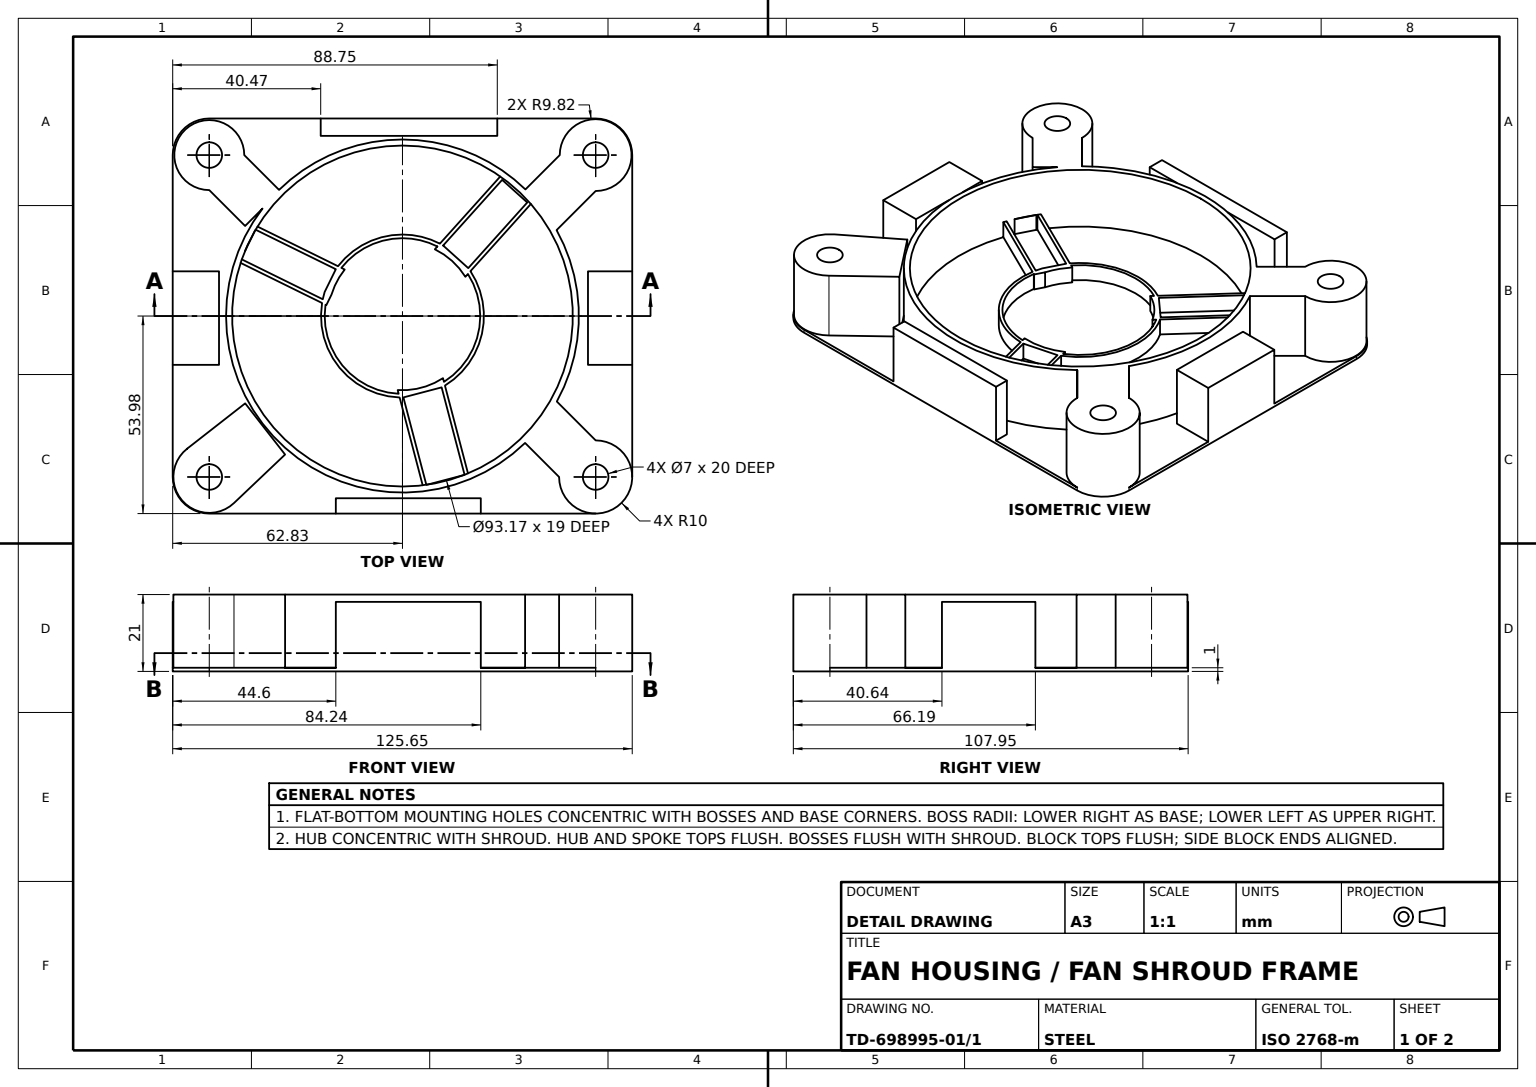
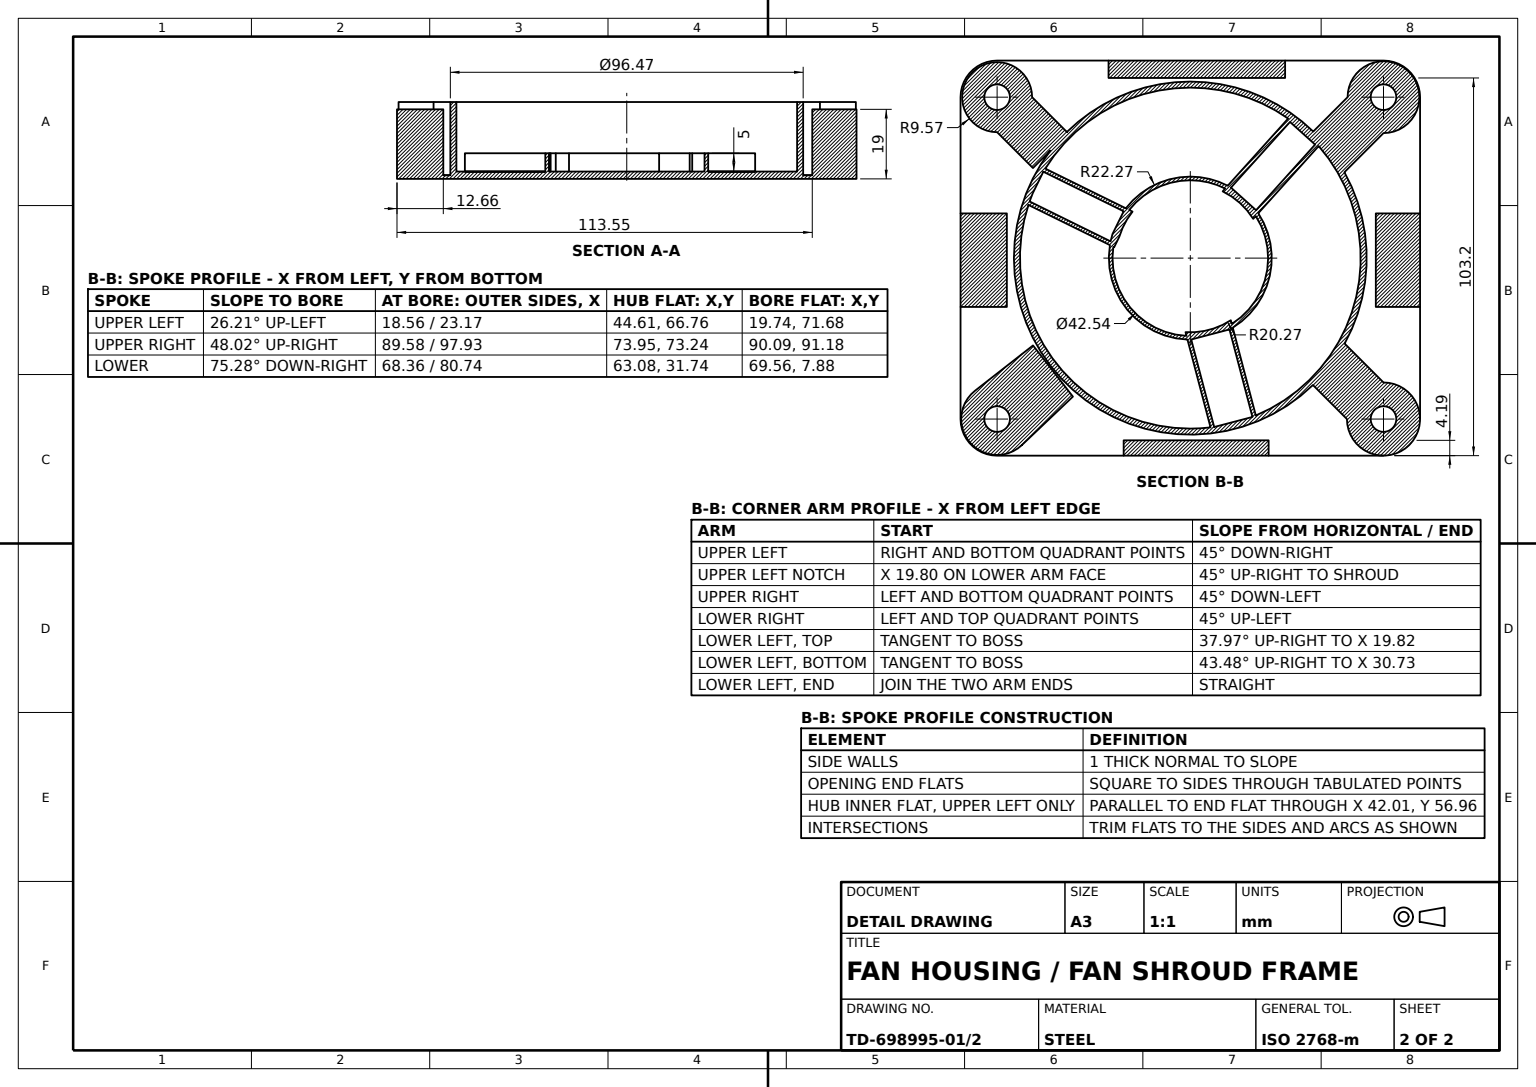
solid
v1 (0,7,-21.270645)
v2 (0,2,-21.270645)
e1 v1 v2 LINE
v3 (9.545019,2,-19.00876)
e2 v3 v2 CIRCLE(AX(P(0,2,0),D(0,1,0),D(0,0,1)),21.270645)
v4 (9.545019,7,-19.00876)
e3 v3 v4 LINE
e4 v4 v1 CIRCLE(AX(P(0,7,0),D(0,1,0),D(0,0,1)),21.270645)
face CYL(AX(P(0,7,0),D(0,-1,0),D(0,0,-1)),21.270645) rev [e1 -e2 e3 e4]
v5 (33.621716,21,-34.589177)
v6 (33.621716,1,-34.589177)
e5 v5 v6 LINE
v7 (43.007539,21,-43.975)
e6 v7 v5 LINE
v8 (43.007539,1,-43.975)
e7 v7 v8 LINE
e8 v8 v6 LINE
face PLANE(AX(P(-0.48373,21,-0.48373),D(0.707106781,0,0.707106781),D(0.707106781,0,-0.707106781))) rev [-e5 -e6 e7 e8]
v9 (52.826203,1,-53.975)
v10 (52.826203,0,-53.975)
e9 v9 v10 LINE
v11 (-52.826203,0,-53.975)
e10 v10 v11 LINE
v12 (-52.826203,1,-53.975)
e11 v12 v11 LINE
v13 (-22.357204,1,-53.975)
e12 v13 v12 LINE
v14 (-22.357204,19,-53.975)
e13 v14 v13 LINE
v15 (25.926841,19,-53.975)
e14 v15 v14 LINE
v16 (25.926841,1,-53.975)
e15 v15 v16 LINE
e16 v9 v16 LINE
face PLANE(AX(P(-52.826203,1,-53.975),D(0,0,1),D(1,0,0))) rev [e9 e10 -e11 -e12 -e13 -e14 e15 -e16]
v17 (-21.7948,2,-4.579116)
v18 (-21.7948,7,-4.579116)
e17 v17 v18 LINE
v19 (-21.281374,7,-6.563897)
e18 v19 v18 CIRCLE(AX(P(0,7,0),D(0,1,0),D(1,0,0)),22.270645)
v20 (-21.281374,2,-6.563897)
e19 v19 v20 LINE
e20 v20 v17 CIRCLE(AX(P(0,2,0),D(0,1,0),D(1,0,0)),22.270645)
face CYL(AX(P(0,7,0),D(0,-1,0),D(0,0,-1)),22.270645) [e17 -e18 e19 e20]
v21 (-32.095624,1,37.844091)
v22 (-46.070336,1,51.098182)
e21 v21 v22 LINE
v23 (-32.095624,21,37.844091)
e22 v23 v21 LINE
v24 (-46.070336,21,51.098182)
e23 v23 v24 LINE
e24 v24 v22 LINE
face PLANE(AX(P(3.696574,21,3.897556),D(0.688151966,0,0.725566587),D(0.725566587,0,-0.688151966))) [-e21 -e22 e23 e24]
v25 (-43.008797,21,23.860209)
v26 (-43.008797,1,23.860209)
e25 v25 v26 LINE
v27 (-58.866196,1,36.235495)
e26 v27 v26 LINE
v28 (-58.866196,21,36.235495)
e27 v28 v27 LINE
e28 v28 v25 LINE
face PLANE(AX(P(-4.706752,21,-6.031121),D(-0.615233142,0,-0.788345217),D(-0.788345217,0,0.615233142))) [e25 -e26 -e27 e28]
v29 (-1.307728,7,20.228418)
v30 (-1.307728,2,20.228418)
e29 v29 v30 LINE
v31 (-1.040622,2,21.245175)
e30 v30 v31 LINE
v32 (-1.040622,7,21.245175)
e31 v31 v32 LINE
e32 v29 v32 LINE
face PLANE(AX(P(-6.194325,7,1.627275),D(0.967182465,0,-0.254082822),D(-0.254082822,0,-0.967182465))) rev [e29 e30 e31 -e32]
v33 (-43.937779,7,-15.47732)
e33 v18 v33 LINE
v34 (-43.937779,2,-15.47732)
e34 v17 v34 LINE
e35 v33 v34 LINE
face PLANE(AX(P(-2.435731,7,4.94892),D(-0.441587655,0,0.897218113),D(0.897218113,0,0.441587655))) rev [-e33 -e17 e34 -e35]
v35 (-40.168907,7,-23.590988)
v36 (-40.168907,2,-23.590988)
e36 v35 v36 LINE
v37 (-18.218296,2,-12.787462)
e37 v37 v36 LINE
v38 (-18.218296,7,-12.787462)
e38 v38 v37 LINE
e39 v38 v35 LINE
face PLANE(AX(P(1.513837,7,-3.075815),D(-0.441587655,0,0.897218113),D(0.897218113,0,0.441587655))) [e36 -e37 -e38 e39]
v39 (-62.826203,1,13.339172)
v40 (-62.826203,1,43.975)
e40 v39 v40 LINE
v41 (-52.826203,1,53.975)
e41 v40 v41 CIRCLE(AX(P(-52.826203,1,43.975),D(0,1,0),D(0,0,1)),10)
v42 (-18.223939,1,53.975)
e42 v41 v42 LINE
v43 (-18.223939,1,49.787051)
e43 v43 v42 LINE
v44 (21.417826,1,49.787051)
e44 v44 v43 LINE
v45 (21.417826,1,53.975)
e45 v45 v44 LINE
v46 (52.826203,1,53.975)
e46 v45 v46 LINE
v47 (42.826203,1,43.975)
e47 v47 v46 CIRCLE(AX(P(52.826203,1,43.975),D(0,1,0),D(0,0,1)),10)
v48 (33.529642,1,34.678439)
e48 v47 v48 LINE
v49 (-38.265553,1,-29.369685)
e49 v49 v48 CIRCLE(AX(P(0,1,0),D(0,1,0),D(0,0,1)),48.237237)
v50 (-43.027328,1,-24.60791)
e50 v50 v49 LINE
v51 (-52.826203,1,-34.406784)
e51 v51 v50 LINE
v52 (-52.826203,1,-53.543216)
e52 v52 v51 CIRCLE(AX(P(-52.826203,1,-43.975),D(0,1,0),D(0,0,1)),9.568216)
v53 (-43.257987,1,-43.975)
e53 v53 v52 CIRCLE(AX(P(-52.826203,1,-43.975),D(0,1,0),D(0,0,1)),9.568216)
v54 (-33.748486,1,-34.465499)
e54 v53 v54 LINE
v55 (0,1,-48.237237)
e55 v55 v54 CIRCLE(AX(P(0,1,0),D(0,1,0),D(0,0,1)),48.237237)
e56 v6 v55 CIRCLE(AX(P(0,1,0),D(0,1,0),D(0,0,1)),48.237237)
v56 (52.826203,1,-53.793663)
e57 v56 v8 CIRCLE(AX(P(52.826203,1,-43.975),D(0,1,0),D(0,0,1)),9.818663)
v57 (52.826203,1,-34.156337)
e58 v57 v56 CIRCLE(AX(P(52.826203,1,-43.975),D(0,1,0),D(0,0,1)),9.818663)
v58 (42.141556,1,-23.47169)
e59 v57 v58 LINE
v59 (42.20629,1,23.355087)
e60 v59 v58 CIRCLE(AX(P(0,1,0),D(0,1,0),D(0,0,1)),48.237237)
v60 (52.826203,1,33.975)
e61 v60 v59 LINE
v61 (62.826203,1,43.975)
e62 v61 v60 CIRCLE(AX(P(52.826203,1,43.975),D(0,1,0),D(0,0,1)),10)
v62 (62.826203,1,13.339172)
e63 v61 v62 LINE
v63 (50.726429,1,13.339172)
e64 v63 v62 LINE
v64 (50.726429,1,-12.211918)
e65 v64 v63 LINE
v65 (62.826203,1,-12.211918)
e66 v65 v64 LINE
v66 (62.826203,1,-43.975)
e67 v65 v66 LINE
e68 v66 v9 CIRCLE(AX(P(52.826203,1,-43.975),D(0,1,0),D(0,0,1)),10)
v67 (25.926841,1,-49.223424)
e69 v67 v16 LINE
v68 (-22.357204,1,-49.223424)
e70 v68 v67 LINE
e71 v13 v68 LINE
v69 (-62.826203,1,-43.975)
e72 v12 v69 CIRCLE(AX(P(-52.826203,1,-43.975),D(0,1,0),D(0,0,-1)),10)
v70 (-62.826203,1,-12.211918)
e73 v69 v70 LINE
v71 (-50.162802,1,-12.211918)
e74 v71 v70 LINE
v72 (-50.162802,1,13.339172)
e75 v72 v71 LINE
e76 v39 v72 LINE
e77 v27 v22 CIRCLE(AX(P(-52.826203,1,43.975),D(0,1,0),D(0,0,1)),9.817406)
e78 v26 v21 LINE
face PLANE(AX(P(52.826203,1,43.975),D(0,-1,0),D(0,0,-1))) rev [e40 e41 e42 -e43 -e44 -e45 e46 -e47 e48 -e49 -e50 -e51 -e52 -e53 e54 -e55 -e56 -e8 -e57 -e58 e59 -e60 -e61 -e62 e63 -e64 -e65 -e66 e67 e68 e16 -e69 -e70 -e71 e12 e72 e73 -e74 -e75 -e76] [-e77 e26 e78 e21]
v73 (-52.826203,1,47.475)
v74 (-52.826203,1,40.475)
e79 v73 v74 CIRCLE(AX(P(-52.826203,1,43.975),D(0,1,0),D(0,0,1)),3.5)
e80 v74 v73 CIRCLE(AX(P(-52.826203,1,43.975),D(0,1,0),D(0,0,1)),3.5)
face PLANE(AX(P(52.826203,1,43.975),D(0,-1,0),D(0,0,-1))) rev [e79 e80]
v75 (52.826203,1,40.475)
v76 (52.826203,1,47.475)
e81 v75 v76 CIRCLE(AX(P(52.826203,1,43.975),D(0,1,0),D(0,0,1)),3.5)
v77 (52.826203,21,40.475)
e82 v77 v75 LINE
v78 (52.826203,21,47.475)
e83 v77 v78 CIRCLE(AX(P(52.826203,21,43.975),D(0,1,0),D(0,0,1)),3.5)
e84 v78 v76 LINE
face CYL(AX(P(52.826203,21,43.975),D(0,-1,0),D(0,0,-1)),3.5) rev [-e81 -e82 e83 e84]
v79 (11.080922,7,16.973868)
v80 (11.080922,2,16.973868)
e85 v79 v80 LINE
e86 v30 v80 CIRCLE(AX(P(0,2,0),D(0,1,0),D(1,0,0)),20.270645)
e87 v29 v79 CIRCLE(AX(P(0,7,0),D(0,1,0),D(1,0,0)),20.270645)
face CYL(AX(P(0,7,0),D(0,-1,0),D(0,0,-1)),20.270645) rev [e85 -e86 -e29 e87]
v81 (-40.311639,2,-23.346255)
e88 v36 v81 CIRCLE(AX(P(0,2,0),D(0,1,0),D(0,0,1)),46.584073)
v82 (-39.651388,7,-24.450834)
e89 v35 v82 CIRCLE(AX(P(0,7,0),D(0,-1,0),D(0,0,1)),46.584073)
v83 (-39.651388,2,-24.450834)
e90 v83 v82 LINE
v84 (0,2,-46.584073)
e91 v84 v83 CIRCLE(AX(P(0,2,0),D(0,1,0),D(0,0,1)),46.584073)
v85 (0,21,-46.584073)
e92 v84 v85 LINE
v86 (0,21,46.584073)
e93 v85 v86 CIRCLE(AX(P(0,21,0),D(0,1,0),D(0,0,1)),46.584073)
v87 (0,2,46.584073)
e94 v87 v86 LINE
v88 (-44.262515,2,-14.52259)
e95 v88 v87 CIRCLE(AX(P(0,2,0),D(0,1,0),D(0,0,1)),46.584073)
v89 (-44.262515,7,-14.52259)
e96 v88 v89 LINE
e97 v89 v33 CIRCLE(AX(P(0,7,0),D(0,-1,0),D(0,0,1)),46.584073)
v90 (-43.08972,2,-17.701747)
e98 v90 v34 CIRCLE(AX(P(0,2,0),D(0,1,0),D(0,0,1)),46.584073)
v91 (-43.08972,7,-17.701747)
e99 v91 v90 LINE
v92 (-40.311639,7,-23.346255)
e100 v91 v92 CIRCLE(AX(P(0,7,0),D(0,-1,0),D(0,0,1)),46.584073)
e101 v92 v81 LINE
face CYL(AX(P(0,2,0),D(0,1,0),D(0,0,1)),46.584073) rev [-e88 -e36 e89 -e90 -e91 e92 e93 -e94 -e95 e96 e97 e35 -e98 -e99 e100 e101]
v93 (18.590913,2,-12.262119)
v94 (18.590913,7,-12.262119)
e102 v93 v94 LINE
v95 (35.107613,2,-30.619134)
e103 v93 v95 LINE
v96 (35.107613,7,-30.619134)
e104 v95 v96 LINE
e105 v94 v96 LINE
face PLANE(AX(P(4.176783,7,3.758055),D(-0.743387039,0,-0.668861503),D(-0.668861503,0,0.743387039))) rev [-e102 e103 e104 -e105]
v97 (17.203804,7,-10.720456)
v98 (17.203804,2,-10.720456)
e106 v97 v98 LINE
v99 (17.898585,2,-11.49265)
e107 v98 v99 LINE
v100 (17.898585,7,-11.49265)
e108 v99 v100 LINE
e109 v97 v100 LINE
face PLANE(AX(P(4.176783,7,3.758055),D(-0.743387039,0,-0.668861503),D(-0.668861503,0,0.743387039))) rev [e106 e107 e108 -e109]
v101 (10.237348,2,-19.778229)
v102 (10.237348,7,-19.778229)
e110 v101 v102 LINE
v103 (0,2,-22.270645)
e111 v101 v103 CIRCLE(AX(P(0,2,0),D(0,1,0),D(1,0,0)),22.270645)
v104 (0,7,-22.270645)
e112 v104 v103 LINE
e113 v102 v104 CIRCLE(AX(P(0,7,0),D(0,1,0),D(1,0,0)),22.270645)
face CYL(AX(P(0,7,0),D(0,-1,0),D(0,0,-1)),22.270645) [-e110 e111 -e112 -e113]
v105 (-43.027328,21,-24.60791)
e114 v105 v50 LINE
v106 (-52.826203,21,-34.406784)
e115 v106 v105 LINE
e116 v106 v51 LINE
face PLANE(AX(P(-9.209709,21,9.209709),D(0.707106781,0,-0.707106781),D(-0.707106781,0,-0.707106781))) rev [-e114 -e115 e116 e51]
v107 (-21.984596,7,-3.557972)
e117 v107 v89 LINE
v108 (-0.774768,7,22.257164)
e118 v107 v108 CIRCLE(AX(P(0,7,0),D(0,1,0),D(1,0,0)),22.270645)
v109 (5.529493,7,46.254735)
e119 v108 v109 LINE
v110 (6.529144,7,46.124247)
e120 v110 v109 CIRCLE(AX(P(0,7,0),D(0,-1,0),D(0,0,1)),46.584073)
v111 (0.254083,7,22.237827)
e121 v111 v110 LINE
v112 (10.708369,7,19.491443)
e122 v111 v112 LINE
v113 (16.98343,7,43.377863)
e123 v112 v113 LINE
v114 (17.918143,7,43.000186)
e124 v114 v113 CIRCLE(AX(P(0,7,0),D(0,-1,0),D(0,0,1)),46.584073)
v115 (11.613882,7,19.002615)
e125 v115 v114 LINE
e126 v115 v94 CIRCLE(AX(P(0,7,0),D(0,1,0),D(1,0,0)),22.270645)
v116 (26.754047,7,-38.135243)
e127 v116 v96 CIRCLE(AX(P(0,7,0),D(0,-1,0),D(0,0,1)),46.584073)
e128 v102 v116 LINE
v117 (-17.627231,7,-13.611111)
e129 v104 v117 CIRCLE(AX(P(0,7,0),D(0,1,0),D(1,0,0)),22.270645)
e130 v117 v82 LINE
e131 v19 v38 LINE
v118 (-15.792502,7,-12.708105)
v119 (-19.415279,7,-5.826317)
e132 v118 v119 CIRCLE(AX(P(0,7,0),D(0,1,0),D(1,0,0)),20.270645)
v120 (-16.710846,7,-13.16009)
e133 v118 v120 LINE
e134 v1 v120 CIRCLE(AX(P(0,7,0),D(0,1,0),D(0,0,1)),21.270645)
v121 (8.850238,7,-18.236566)
e135 v121 v4 LINE
e136 v97 v121 CIRCLE(AX(P(0,7,0),D(0,1,0),D(1,0,0)),20.270645)
v122 (11.348029,7,17.990625)
e137 v122 v100 CIRCLE(AX(P(0,7,0),D(0,1,0),D(0,0,1)),21.270645)
e138 v79 v122 LINE
v123 (-21.044247,7,-3.095157)
e139 v123 v32 CIRCLE(AX(P(0,7,0),D(0,1,0),D(0,0,1)),21.270645)
v124 (-20.815015,7,-2.982334)
e140 v124 v123 LINE
e141 v124 v119 LINE
v125 (27.258813,7,-37.201174)
v126 (34.125605,7,-31.022787)
e142 v125 v126 LINE
v127 (17.989939,7,-13.089261)
e143 v127 v126 LINE
v128 (11.123147,7,-19.267648)
e144 v128 v127 LINE
e145 v128 v125 LINE
face PLANE(AX(P(0,7,0),D(0,1,0),D(0,0,1))) [-e117 e118 e119 -e120 -e121 e122 e123 -e124 -e125 e126 e105 -e127 -e128 e113 e129 e130 -e89 -e39 -e131 e18 e33 -e97] [-e132 e133 -e134 -e4 -e135 -e136 e109 -e137 -e138 -e87 e32 -e139 -e140 e141] [e142 -e143 -e144 e145]
v129 (11.123147,2,-19.267648)
e146 v128 v129 LINE
v130 (27.258813,2,-37.201174)
e147 v129 v130 LINE
e148 v125 v130 LINE
face PLANE(AX(P(-3.433396,7,-3.089193),D(-0.743387039,0,-0.668861503),D(-0.668861503,0,0.743387039))) rev [-e145 e146 e147 -e148]
v131 (-17.627231,2,-13.611111)
e149 v103 v131 CIRCLE(AX(P(0,2,0),D(0,1,0),D(1,0,0)),22.270645)
v132 (26.754047,2,-38.135243)
e150 v101 v132 LINE
e151 v132 v84 CIRCLE(AX(P(0,2,0),D(0,1,0),D(0,0,1)),46.584073)
e152 v131 v83 LINE
face PLANE(AX(P(0,2,0),D(0,1,0),D(0,0,1))) [-e149 -e111 e150 e151 e91 -e152]
v133 (52.826203,21,-34.156337)
e153 v133 v57 LINE
v134 (42.141556,21,-23.47169)
e154 v133 v134 LINE
e155 v134 v58 LINE
face PLANE(AX(P(9.334933,21,9.334933),D(0.707106781,0,0.707106781),D(0.707106781,0,-0.707106781))) [-e153 e154 e155 -e59]
e156 v20 v37 LINE
face PLANE(AX(P(-19.732132,7,-9.711647),D(-0.897218113,0,-0.441587655),D(-0.441587655,0,0.897218113))) [e131 e38 -e156 -e19]
v135 (17.989939,2,-13.089261)
e157 v129 v135 LINE
v136 (34.125605,2,-31.022787)
e158 v135 v136 LINE
e159 v130 v136 LINE
face PLANE(AX(P(0,2,0),D(0,1,0),D(0,0,1))) [e157 e158 -e159 -e147]
e160 v126 v136 LINE
face PLANE(AX(P(30.692209,7,-34.11198),D(0.668861503,0,-0.743387039),D(-0.743387039,0,-0.668861503))) rev [-e160 -e142 e148 e159]
v137 (0.254083,2,22.237827)
v138 (6.529144,2,46.124247)
e161 v137 v138 LINE
e162 v137 v111 LINE
e163 v110 v138 LINE
face PLANE(AX(P(-5.227143,7,1.373192),D(0.967182465,0,-0.254082822),D(-0.254082822,0,-0.967182465))) [-e161 e162 e121 e163]
v139 (8.850238,2,-18.236566)
e164 v98 v139 CIRCLE(AX(P(0,2,0),D(0,1,0),D(1,0,0)),20.270645)
e165 v121 v139 LINE
face CYL(AX(P(0,7,0),D(0,-1,0),D(0,0,-1)),20.270645) rev [-e164 -e106 e136 e165]
e166 v76 v75 CIRCLE(AX(P(52.826203,1,43.975),D(0,1,0),D(0,0,1)),3.5)
face PLANE(AX(P(52.826203,1,43.975),D(0,-1,0),D(0,0,-1))) rev [e166 e81]
v140 (52.826203,1,-47.475)
v141 (52.826203,1,-40.475)
e167 v140 v141 CIRCLE(AX(P(52.826203,1,-43.975),D(0,1,0),D(0,0,1)),3.5)
v142 (52.826203,21,-47.475)
e168 v142 v140 LINE
v143 (52.826203,21,-40.475)
e169 v142 v143 CIRCLE(AX(P(52.826203,21,-43.975),D(0,1,0),D(0,0,1)),3.5)
e170 v143 v141 LINE
face CYL(AX(P(52.826203,21,-43.975),D(0,-1,0),D(0,0,-1)),3.5) rev [-e167 -e168 e169 e170]
v144 (-18.223939,19,49.787051)
e171 v144 v43 LINE
v145 (-18.223939,19,53.975)
e172 v145 v42 LINE
e173 v144 v145 LINE
face PLANE(AX(P(-18.223939,19,53.975),D(1,0,0),D(0,0,-1))) rev [e171 e43 -e172 -e173]
v146 (11.348029,2,17.990625)
e174 v146 v122 LINE
e175 v80 v146 LINE
face PLANE(AX(P(6.194325,7,-1.627275),D(0.967182465,0,-0.254082822),D(-0.254082822,0,-0.967182465))) [e138 -e174 -e175 -e85]
e176 v25 v23 LINE
face PLANE(AX(P(-38.302045,21,29.89133),D(0.788345217,0,-0.615233142),D(-0.615233142,0,-0.788345217))) [e176 e22 -e78 -e25]
v147 (-38.265553,21,-29.369685)
e177 v105 v147 LINE
e178 v147 v49 LINE
face PLANE(AX(P(-33.817619,21,-33.817619),D(-0.707106781,0,-0.707106781),D(-0.707106781,0,0.707106781))) rev [-e177 e114 e50 -e178]
v148 (50.726429,19,-12.211918)
v149 (50.726429,19,13.339172)
e179 v148 v149 LINE
e180 v148 v64 LINE
e181 v149 v63 LINE
face PLANE(AX(P(50.726429,19,-12.211918),D(1,0,0),D(0,0,-1))) rev [-e179 e180 e65 -e181]
v150 (-21.984596,2,-3.557972)
e182 v150 v88 LINE
v151 (5.529493,2,46.254735)
e183 v87 v151 CIRCLE(AX(P(0,2,0),D(0,1,0),D(0,0,1)),46.584073)
v152 (-0.774768,2,22.257164)
e184 v152 v151 LINE
e185 v150 v152 CIRCLE(AX(P(0,2,0),D(0,1,0),D(1,0,0)),22.270645)
face PLANE(AX(P(0,2,0),D(0,1,0),D(0,0,1))) [e182 e95 e183 -e184 -e185]
v153 (-43.257987,21,-43.975)
e186 v153 v53 LINE
v154 (-33.748486,21,-34.465499)
e187 v153 v154 LINE
e188 v154 v54 LINE
face PLANE(AX(P(0.358506,21,-0.358506),D(0.707106781,0,-0.707106781),D(-0.707106781,0,-0.707106781))) [-e54 -e186 e187 e188]
v155 (42.826203,21,43.975)
v156 (33.529642,21,34.678439)
e189 v155 v156 LINE
e190 v156 v48 LINE
e191 v155 v47 LINE
face PLANE(AX(P(-0.574399,21,0.574399),D(-0.707106781,0,0.707106781),D(0.707106781,0,0.707106781))) [e189 e190 -e48 -e191]
v157 (10.708369,2,19.491443)
v158 (16.98343,2,43.377863)
e192 v157 v158 LINE
e193 v113 v158 LINE
e194 v157 v112 LINE
face PLANE(AX(P(5.227143,7,-1.373192),D(0.967182465,0,-0.254082822),D(-0.254082822,0,-0.967182465))) rev [e192 -e193 -e123 -e194]
v159 (62.826203,19,13.339172)
e195 v149 v159 LINE
v160 (62.826203,19,-12.211918)
e196 v159 v160 LINE
e197 v160 v148 LINE
face PLANE(AX(P(0,19,0),D(0,-1,0),D(0,0,-1))) rev [e179 e195 e196 e197]
v161 (52.826203,21,33.975)
e198 v161 v60 LINE
e199 v155 v161 CIRCLE(AX(P(52.826203,21,43.975),D(0,1,0),D(0,0,1)),10)
v162 (52.826203,0,53.975)
e200 v46 v162 LINE
v163 (62.826203,0,43.975)
e201 v162 v163 CIRCLE(AX(P(52.826203,0,43.975),D(0,1,0),D(0,0,-1)),10)
e202 v61 v163 LINE
face CYL(AX(P(52.826203,1,43.975),D(0,-1,0),D(0,0,-1)),10) [e62 -e198 -e199 e191 e47 e200 e201 -e202]
e203 v143 v142 CIRCLE(AX(P(52.826203,21,-43.975),D(0,1,0),D(0,0,1)),3.5)
v164 (42.20629,21,23.355087)
e204 v161 v164 LINE
e205 v164 v134 CIRCLE(AX(P(0,21,0),D(0,1,0),D(0,0,1)),48.237237)
v165 (52.826203,21,-53.793663)
e206 v133 v165 CIRCLE(AX(P(52.826203,21,-43.975),D(0,1,0),D(0,0,1)),9.818663)
e207 v165 v7 CIRCLE(AX(P(52.826203,21,-43.975),D(0,1,0),D(0,0,1)),9.818663)
v166 (0,21,-48.237237)
e208 v5 v166 CIRCLE(AX(P(0,21,0),D(0,1,0),D(0,0,1)),48.237237)
e209 v166 v154 CIRCLE(AX(P(0,21,0),D(0,1,0),D(0,0,1)),48.237237)
v167 (-52.826203,21,-53.543216)
e210 v153 v167 CIRCLE(AX(P(-52.826203,21,-43.975),D(0,1,0),D(0,0,1)),9.568216)
e211 v167 v106 CIRCLE(AX(P(-52.826203,21,-43.975),D(0,1,0),D(0,0,1)),9.568216)
e212 v147 v156 CIRCLE(AX(P(0,21,0),D(0,1,0),D(0,0,1)),48.237237)
v168 (-52.826203,21,-40.475)
v169 (-52.826203,21,-47.475)
e213 v168 v169 CIRCLE(AX(P(-52.826203,21,-43.975),D(0,1,0),D(0,0,1)),3.5)
e214 v169 v168 CIRCLE(AX(P(-52.826203,21,-43.975),D(0,1,0),D(0,0,1)),3.5)
e215 v78 v77 CIRCLE(AX(P(52.826203,21,43.975),D(0,1,0),D(0,0,1)),3.5)
e216 v86 v85 CIRCLE(AX(P(0,21,0),D(0,1,0),D(0,0,1)),46.584073)
face PLANE(AX(P(0,21,0),D(0,1,0),D(0,0,1))) [-e203 -e169] [e199 e204 e205 -e154 e206 e207 e6 e208 e209 -e187 e210 e211 e115 e177 e212 -e189] [-e213 -e214] [-e215 -e83] [-e93 -e216]
v170 (-62.826203,19,13.339172)
e217 v170 v39 LINE
v171 (-62.826203,19,-12.211918)
e218 v171 v170 LINE
e219 v171 v70 LINE
v172 (-62.826203,0,-43.975)
e220 v69 v172 LINE
v173 (-62.826203,0,43.975)
e221 v172 v173 LINE
e222 v40 v173 LINE
face PLANE(AX(P(-62.826203,1,-43.975),D(1,0,0),D(0,0,-1))) rev [-e40 -e217 -e218 e219 -e73 e220 e221 -e222]
e223 v90 v81 LINE
e224 v91 v92 LINE
face PLANE(AX(P(-41.70068,7,-20.524001),D(-0.897218113,0,-0.441587655),D(-0.441587655,0,0.897218113))) rev [e99 e223 -e101 -e224]
face CYL(AX(P(0,21,0),D(0,-1,0),D(0,0,-1)),48.237237) [e49 -e190 -e212 e178]
e225 v127 v135 LINE
face PLANE(AX(P(3.433396,7,3.089193),D(-0.743387039,0,-0.668861503),D(-0.668861503,0,0.743387039))) [e160 -e158 -e225 e143]
e226 v11 v172 CIRCLE(AX(P(-52.826203,0,-43.975),D(0,1,0),D(0,0,-1)),10)
face CYL(AX(P(-52.826203,1,-43.975),D(0,-1,0),D(0,0,-1)),10) [e11 e226 -e220 -e72]
e227 v160 v65 LINE
e228 v159 v62 LINE
v174 (62.826203,0,-43.975)
e229 v163 v174 LINE
e230 v66 v174 LINE
face PLANE(AX(P(62.826203,1,-43.975),D(-1,0,0),D(0,0,1))) rev [-e227 -e196 e228 -e63 e202 e229 -e230 -e67]
v175 (-50.162802,19,-12.211918)
e231 v175 v71 LINE
e232 v175 v171 LINE
face PLANE(AX(P(-62.826203,19,-12.211918),D(0,0,1),D(1,0,0))) rev [e231 e74 -e219 -e232]
v176 (21.417826,19,49.787051)
e233 v176 v44 LINE
v177 (21.417826,19,53.975)
e234 v177 v176 LINE
e235 v177 v45 LINE
face PLANE(AX(P(21.417826,19,53.975),D(-1,0,0),D(0,0,1))) rev [e45 -e233 -e234 e235]
face PLANE(AX(P(62.826203,19,-12.211918),D(0,0,1),D(1,0,0))) rev [e66 -e180 -e197 e227]
face PLANE(AX(P(0,2,0),D(0,1,0),D(0,0,1))) [e37 e88 -e223 e98 -e34 -e20 e156]
e236 v165 v56 LINE
face CYL(AX(P(52.826203,21,-43.975),D(0,-1,0),D(0,0,-1)),9.818663) [-e206 e153 e58 -e236]
e237 v176 v144 LINE
face PLANE(AX(P(-18.223939,19,49.787051),D(0,0,1),D(1,0,0))) rev [-e237 e233 e44 -e171]
e238 v146 v99 CIRCLE(AX(P(0,2,0),D(0,1,0),D(0,0,1)),21.270645)
face CYL(AX(P(0,7,0),D(0,-1,0),D(0,0,-1)),21.270645) rev [-e238 e174 e137 -e108]
face CYL(AX(P(52.826203,21,-43.975),D(0,-1,0),D(0,0,-1)),9.818663) [e236 e57 -e7 -e207]
v178 (-52.826203,21,47.475)
e239 v178 v73 LINE
v179 (-52.826203,21,40.475)
e240 v179 v74 LINE
e241 v179 v178 CIRCLE(AX(P(-52.826203,21,43.975),D(0,1,0),D(0,0,1)),3.5)
face CYL(AX(P(-52.826203,21,43.975),D(0,-1,0),D(0,0,-1)),3.5) rev [e239 -e80 -e240 e241]
v180 (-21.044247,2,-3.095157)
e242 v180 v123 LINE
e243 v180 v31 CIRCLE(AX(P(0,2,0),D(0,1,0),D(0,0,1)),21.270645)
face CYL(AX(P(0,7,0),D(0,-1,0),D(0,0,-1)),21.270645) rev [e242 e139 -e31 -e243]
face PLANE(AX(P(0,7,0),D(0,1,0),D(0,0,1))) [-e100 e224]
e244 v131 v117 LINE
face PLANE(AX(P(1.955424,7,-3.973033),D(-0.441587655,0,0.897218113),D(0.897218113,0,0.441587655))) rev [-e244 e152 e90 -e130]
e245 v150 v107 LINE
face PLANE(AX(P(-2.877318,7,5.846138),D(-0.441587655,0,0.897218113),D(0.897218113,0,0.441587655))) [e245 e117 -e96 -e182]
v181 (-15.792502,2,-12.708105)
e246 v118 v181 LINE
v182 (-16.710846,2,-13.16009)
e247 v181 v182 LINE
e248 v182 v120 LINE
face PLANE(AX(P(1.955424,7,-3.973033),D(-0.441587655,0,0.897218113),D(0.897218113,0,0.441587655))) rev [e246 e247 e248 -e133]
face CYL(AX(P(0,7,0),D(0,-1,0),D(0,0,-1)),22.270645) [e112 e149 e244 -e129]
v183 (16.792216,7,43.452242)
v184 (6.732224,7,46.095043)
e249 v183 v184 CIRCLE(AX(P(0,7,0),D(0,-1,0),D(0,0,1)),46.584073)
e250 v184 v183 LINE
face PLANE(AX(P(0,7,0),D(0,1,0),D(0,0,1))) [-e249 -e250]
e251 v152 v108 LINE
face CYL(AX(P(0,7,0),D(0,-1,0),D(0,0,-1)),22.270645) [-e245 e185 e251 -e118]
v185 (-22.357204,19,-49.223424)
e252 v185 v68 LINE
e253 v14 v185 LINE
face PLANE(AX(P(-22.357204,19,-53.975),D(1,0,0),D(0,0,-1))) rev [e13 e71 -e252 -e253]
v186 (-52.826203,1,-47.475)
v187 (-52.826203,1,-40.475)
e254 v186 v187 CIRCLE(AX(P(-52.826203,1,-43.975),D(0,1,0),D(0,0,1)),3.5)
e255 v187 v186 CIRCLE(AX(P(-52.826203,1,-43.975),D(0,1,0),D(0,0,1)),3.5)
face PLANE(AX(P(52.826203,1,43.975),D(0,-1,0),D(0,0,-1))) rev [e254 e255]
e256 v169 v186 LINE
e257 v168 v187 LINE
face CYL(AX(P(-52.826203,21,-43.975),D(0,-1,0),D(0,0,-1)),3.5) rev [-e256 e214 e257 -e254]
v188 (17.918143,2,43.000186)
e258 v188 v95 CIRCLE(AX(P(0,2,0),D(0,1,0),D(0,0,1)),46.584073)
e259 v188 v114 LINE
v189 (16.792216,2,43.452242)
e260 v189 v158 CIRCLE(AX(P(0,2,0),D(0,1,0),D(0,0,1)),46.584073)
e261 v183 v189 LINE
v190 (6.732224,2,46.095043)
e262 v184 v190 LINE
e263 v138 v190 CIRCLE(AX(P(0,2,0),D(0,1,0),D(0,0,1)),46.584073)
e264 v151 v109 LINE
e265 v132 v116 LINE
face CYL(AX(P(0,2,0),D(0,1,0),D(0,0,1)),46.584073) rev [-e104 -e258 e259 e124 e193 -e260 -e261 e249 e262 -e263 -e163 e120 -e264 -e183 e94 e216 -e92 -e151 e265 e127]
v191 (25.926841,19,-49.223424)
e266 v191 v67 LINE
e267 v185 v191 LINE
face PLANE(AX(P(-22.357204,19,-49.223424),D(0,0,-1),D(-1,0,0))) rev [-e266 -e267 e252 e70]
e268 v2 v182 CIRCLE(AX(P(0,2,0),D(0,1,0),D(0,0,1)),21.270645)
face CYL(AX(P(0,7,0),D(0,-1,0),D(0,0,-1)),21.270645) rev [-e1 e134 -e248 -e268]
e269 v166 v55 LINE
face CYL(AX(P(0,21,0),D(0,-1,0),D(0,0,-1)),48.237237) [e56 -e269 -e208 e5]
e270 v190 v189 LINE
face PLANE(AX(P(11.76222,7,44.773642),D(-0.254082822,0,-0.967182465),D(-0.967182465,0,0.254082822))) [-e262 e250 e261 -e270]
v192 (-52.826203,0,53.975)
e271 v192 v162 LINE
e272 v173 v192 CIRCLE(AX(P(-52.826203,0,43.975),D(0,1,0),D(0,0,1)),10)
e273 v174 v10 CIRCLE(AX(P(52.826203,0,-43.975),D(0,1,0),D(0,0,1)),10)
face PLANE(AX(P(52.826203,0,43.975),D(0,-1,0),D(0,0,-1))) [-e201 -e271 -e272 -e221 -e226 -e10 -e273 -e229]
e274 v139 v3 LINE
face PLANE(AX(P(-4.176783,7,-3.758055),D(-0.743387039,0,-0.668861503),D(-0.668861503,0,0.743387039))) [-e274 -e165 e135 -e3]
e275 v41 v192 LINE
face CYL(AX(P(-52.826203,1,43.975),D(0,-1,0),D(0,0,-1)),10) [e272 -e275 -e41 e222]
v193 (-19.415279,2,-5.826317)
e276 v181 v193 CIRCLE(AX(P(0,2,0),D(0,1,0),D(1,0,0)),20.270645)
e277 v119 v193 LINE
face CYL(AX(P(0,7,0),D(0,-1,0),D(0,0,-1)),20.270645) rev [-e276 -e246 e132 e277]
e278 v145 v177 LINE
face PLANE(AX(P(0,19,0),D(0,-1,0),D(0,0,-1))) rev [e173 e278 e234 e237]
v194 (11.613882,2,19.002615)
e279 v194 v115 LINE
e280 v194 v93 CIRCLE(AX(P(0,2,0),D(0,1,0),D(1,0,0)),22.270645)
face CYL(AX(P(0,7,0),D(0,-1,0),D(0,0,-1)),22.270645) [-e126 -e279 e280 e102]
e281 v164 v59 LINE
face CYL(AX(P(0,21,0),D(0,-1,0),D(0,0,-1)),48.237237) [e281 e60 -e155 -e205]
e282 v194 v188 LINE
face PLANE(AX(P(6.194325,7,-1.627275),D(0.967182465,0,-0.254082822),D(-0.254082822,0,-0.967182465))) [-e259 -e282 e279 e125]
e283 v28 v24 CIRCLE(AX(P(-52.826203,21,43.975),D(0,1,0),D(0,0,1)),9.817406)
face CYL(AX(P(-52.826203,21,43.975),D(0,-1,0),D(0,0,-1)),9.817406) [e27 e77 -e24 -e283]
v195 (-50.162802,19,13.339172)
e284 v195 v72 LINE
e285 v170 v195 LINE
face PLANE(AX(P(-62.826203,19,13.339172),D(0,0,-1),D(-1,0,0))) rev [e76 -e284 -e285 e217]
face CYL(AX(P(0,21,0),D(0,-1,0),D(0,0,-1)),48.237237) [-e209 e269 e55 -e188]
e286 v195 v175 LINE
face PLANE(AX(P(0,19,0),D(0,1,0),D(0,0,1))) [e232 e218 e285 e286]
face PLANE(AX(P(-6.194325,7,1.627275),D(0.967182465,0,-0.254082822),D(-0.254082822,0,-0.967182465))) rev [-e251 e184 e264 -e119]
face CYL(AX(P(-52.826203,21,-43.975),D(0,-1,0),D(0,0,-1)),3.5) rev [-e255 -e257 e213 e256]
face PLANE(AX(P(-52.826203,1,53.975),D(0,0,-1),D(-1,0,0))) rev [e172 -e42 e275 e271 -e200 -e46 -e235 -e278]
face PLANE(AX(P(-4.176783,7,-3.758055),D(-0.743387039,0,-0.668861503),D(-0.668861503,0,0.743387039))) [-e265 -e150 e110 e128]
face PLANE(AX(P(9.425601,21,-9.425601),D(-0.707106781,0,0.707106781),D(0.707106781,0,0.707106781))) rev [-e281 -e204 e198 e61]
e287 v191 v15 LINE
face PLANE(AX(P(0,19,0),D(0,1,0),D(0,0,1))) [e287 e14 e253 e267]
e288 v137 v157 LINE
face PLANE(AX(P(5.481226,7,20.864635),D(-0.254082822,0,-0.967182465),D(-0.967182465,0,0.254082822))) rev [-e162 e288 e194 -e122]
e289 v167 v52 LINE
face CYL(AX(P(-52.826203,21,-43.975),D(0,-1,0),D(0,0,-1)),9.568216) [e186 e53 -e289 -e210]
face CYL(AX(P(-52.826203,21,-43.975),D(0,-1,0),D(0,0,-1)),9.568216) [-e211 e289 e52 -e116]
face CYL(AX(P(52.826203,21,43.975),D(0,-1,0),D(0,0,-1)),3.5) rev [-e166 -e84 e215 e82]
face CYL(AX(P(52.826203,1,-43.975),D(0,-1,0),D(0,0,-1)),10) [-e68 e230 e273 -e9]
e290 v141 v140 CIRCLE(AX(P(52.826203,1,-43.975),D(0,1,0),D(0,0,1)),3.5)
face CYL(AX(P(52.826203,21,-43.975),D(0,-1,0),D(0,0,-1)),3.5) rev [-e290 -e170 e203 e168]
e291 v178 v179 CIRCLE(AX(P(-52.826203,21,43.975),D(0,1,0),D(0,0,1)),3.5)
face PLANE(AX(P(0,21,0),D(0,1,0),D(0,0,1))) [-e291 -e241] [-e23 -e176 -e28 e283]
face CYL(AX(P(-52.826203,21,43.975),D(0,-1,0),D(0,0,-1)),3.5) rev [-e79 -e239 e291 e240]
v196 (-20.815015,2,-2.982334)
e292 v124 v196 LINE
e293 v196 v193 LINE
face PLANE(AX(P(-17.937696,7,-8.828472),D(-0.897218113,0,-0.441587655),D(-0.441587655,0,0.897218113))) rev [e292 e293 -e277 -e141]
face PLANE(AX(P(62.826203,19,13.339172),D(0,0,-1),D(-1,0,0))) rev [-e195 e181 e64 -e228]
face PLANE(AX(P(52.826203,1,43.975),D(0,-1,0),D(0,0,-1))) rev [e167 e290]
face PLANE(AX(P(14.556543,7,-16.178455),D(0.668861503,0,-0.743387039),D(-0.743387039,0,-0.668861503))) [e144 e225 -e157 -e146]
e294 v196 v180 LINE
face PLANE(AX(P(0,2,0),D(0,1,0),D(0,0,1))) [-e293 e294 e243 -e30 e86 e175 e238 -e107 e164 e274 e2 e268 -e247 e276]
face PLANE(AX(P(0,2,0),D(0,1,0),D(0,0,1))) [e258 -e103 -e280 e282]
face PLANE(AX(P(-2.877318,7,5.846138),D(-0.441587655,0,0.897218113),D(0.897218113,0,0.441587655))) [e140 -e242 -e294 -e292]
face PLANE(AX(P(0,2,0),D(0,1,0),D(0,0,1))) [e270 e260 -e192 -e288 e161 e263]
face PLANE(AX(P(-50.162802,19,-12.211918),D(-1,0,0),D(0,0,1))) rev [e75 -e231 -e286 e284]
face PLANE(AX(P(25.926841,19,-53.975),D(-1,0,0),D(0,0,1))) rev [-e287 e266 e69 -e15]
